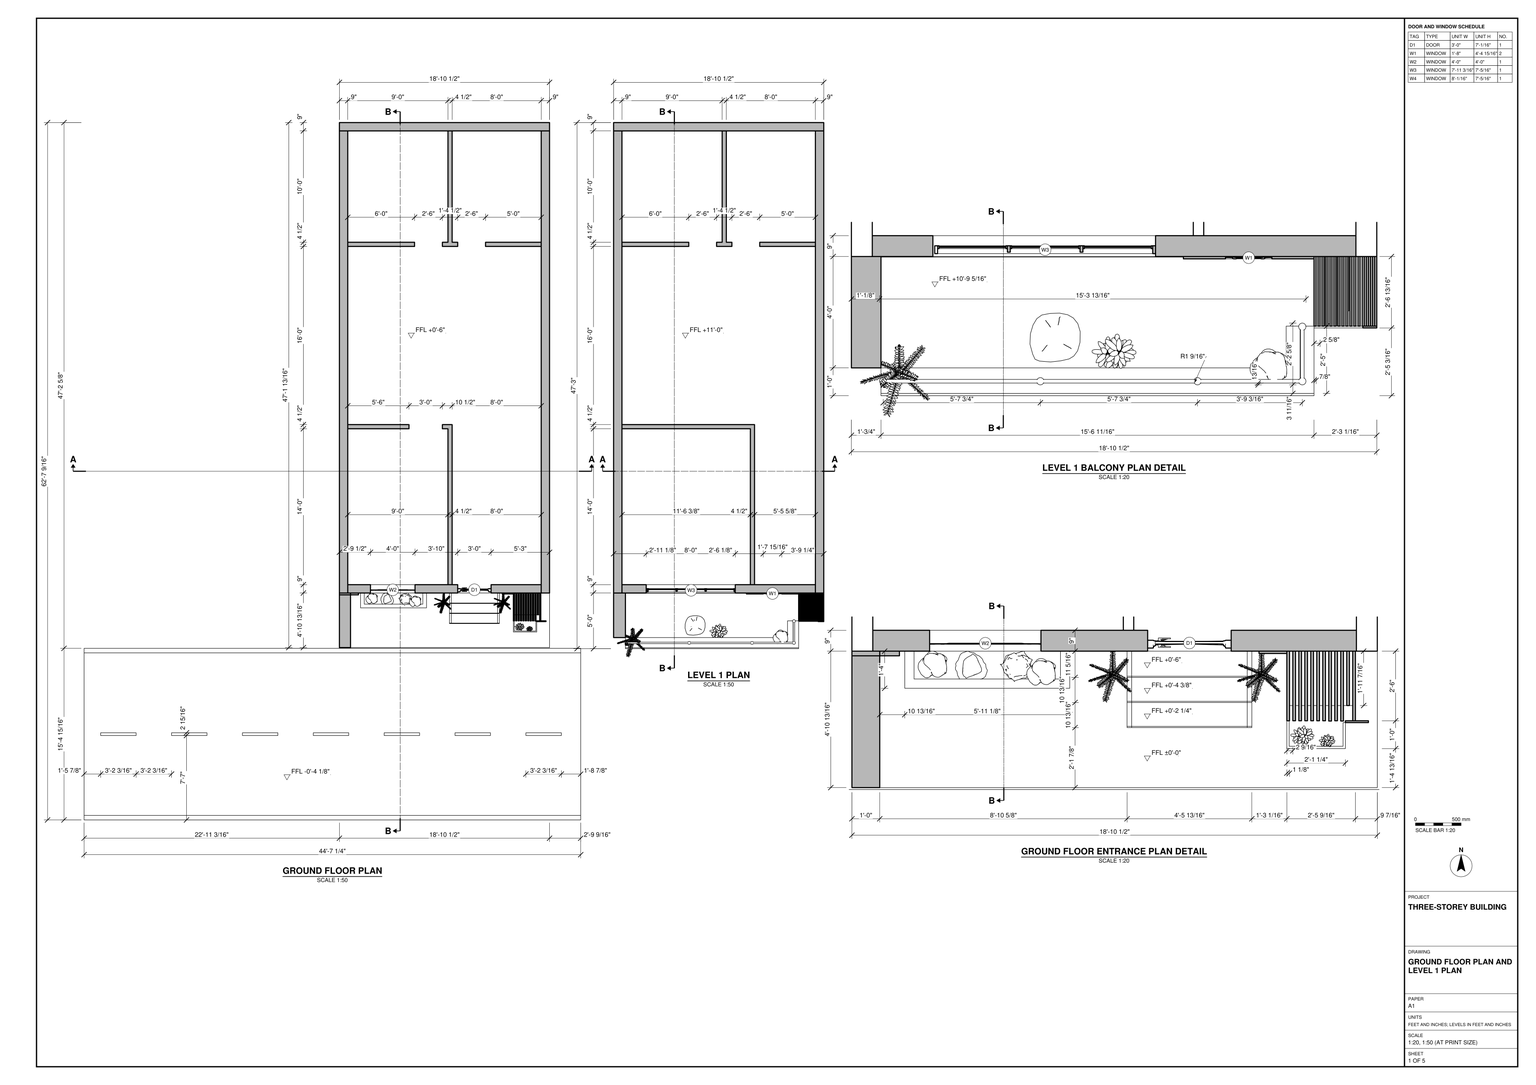
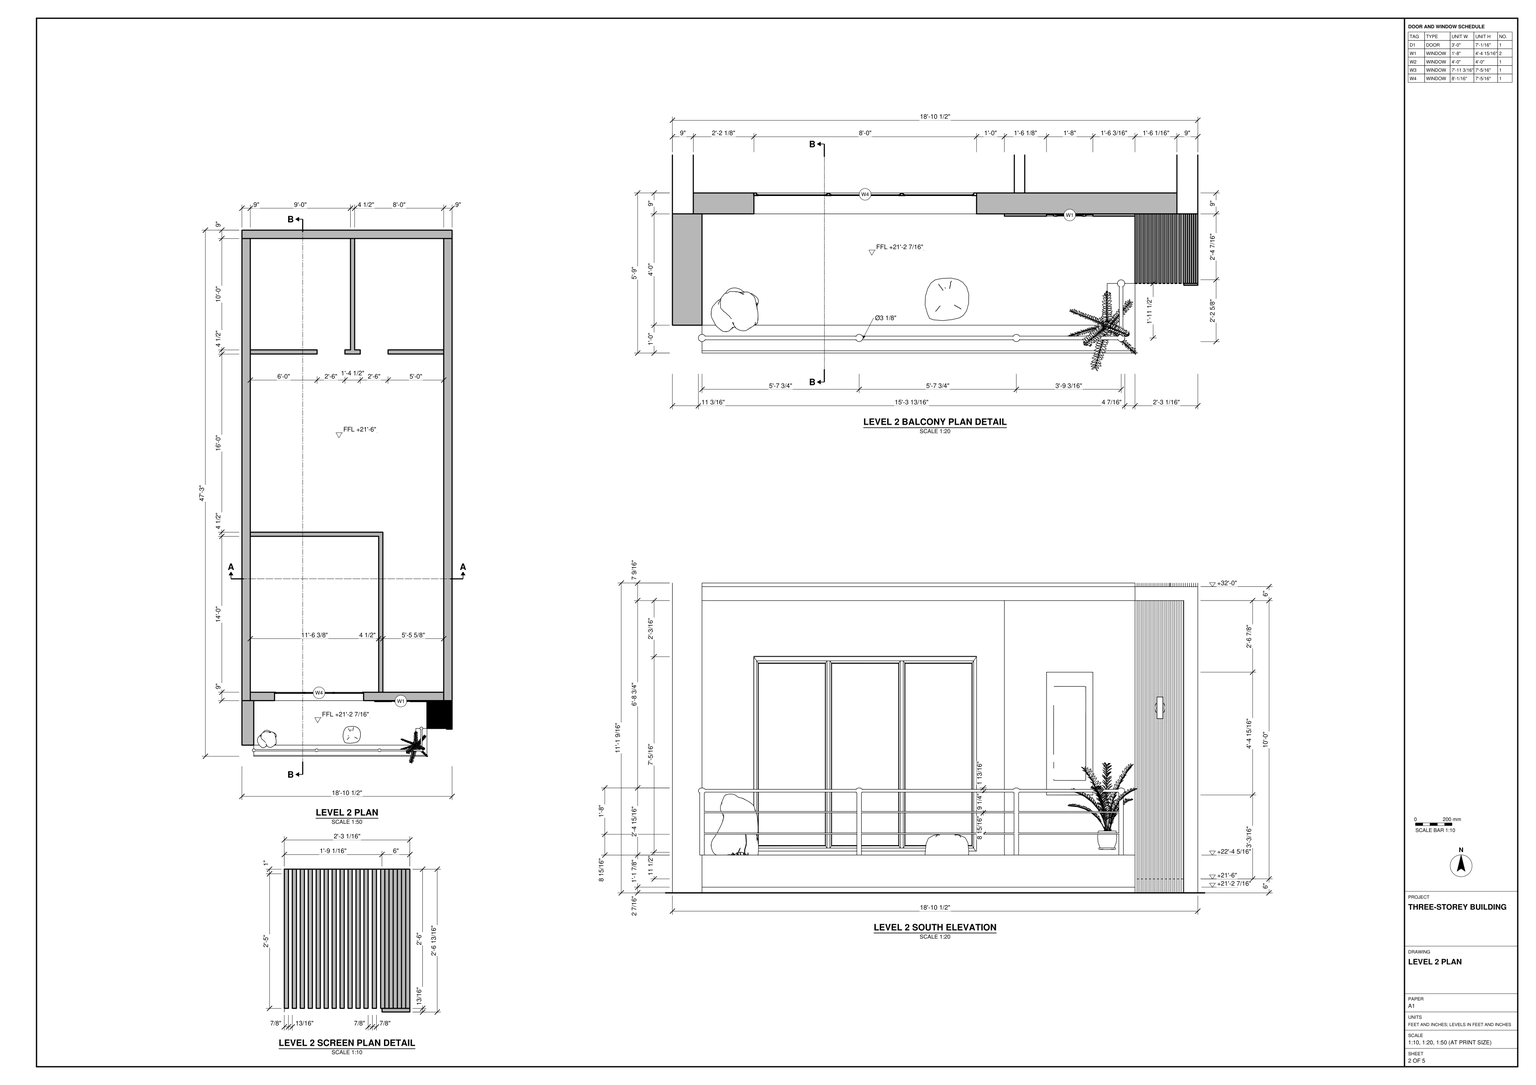
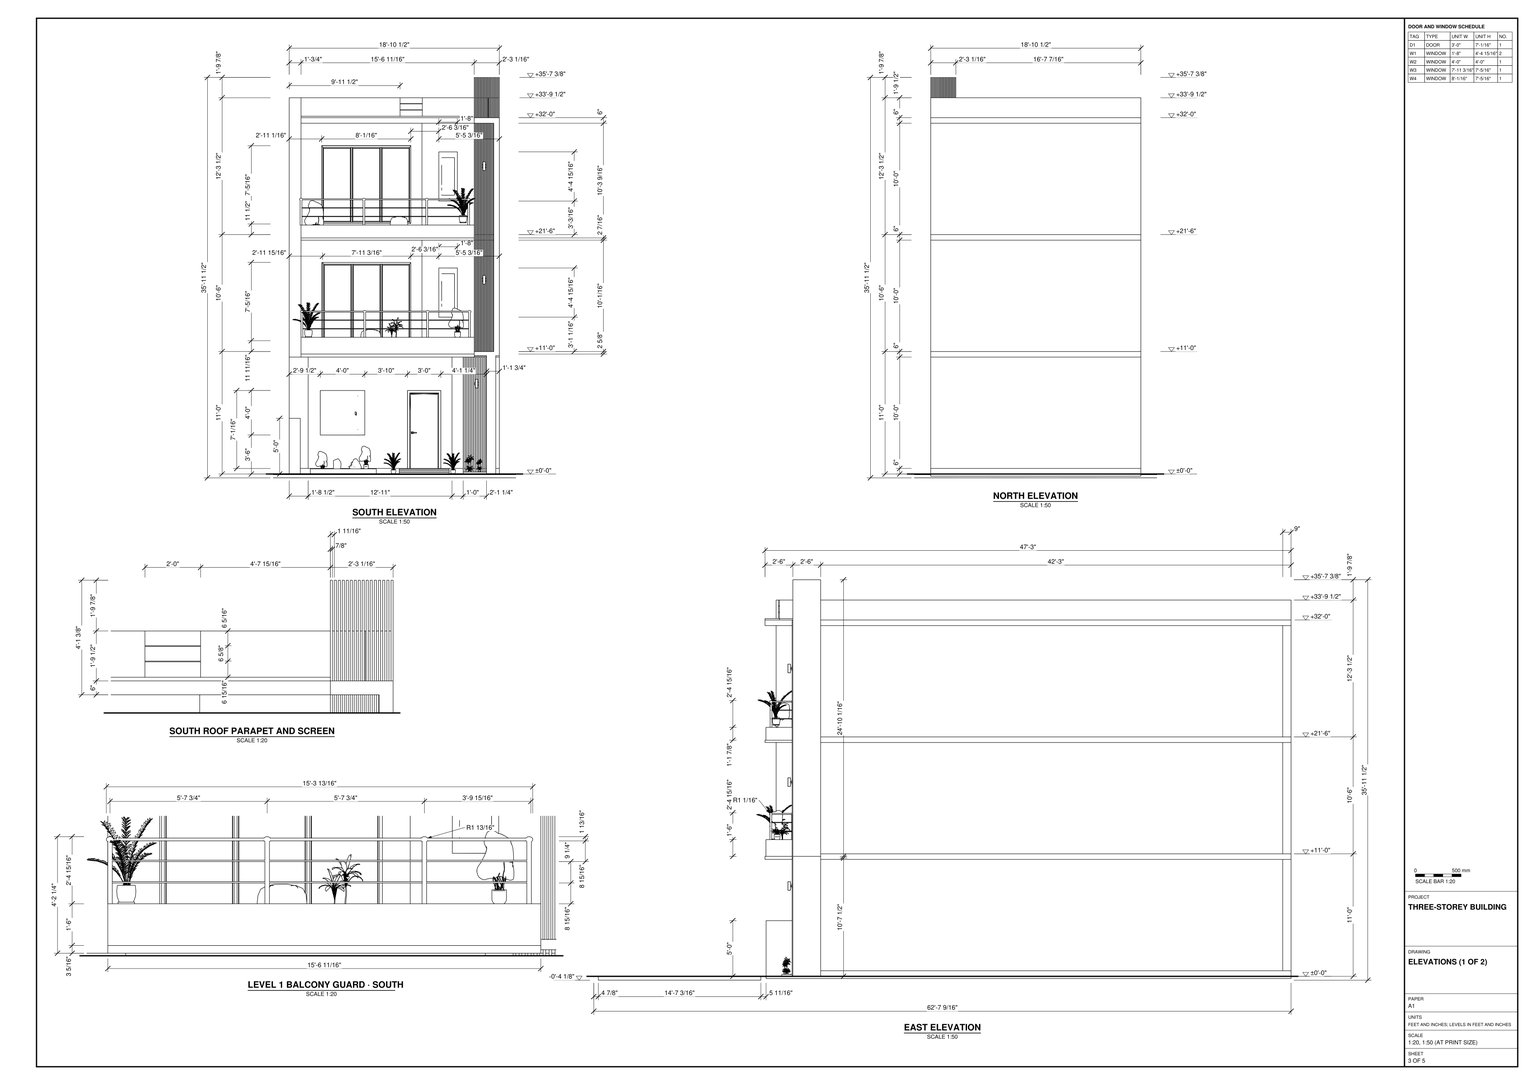
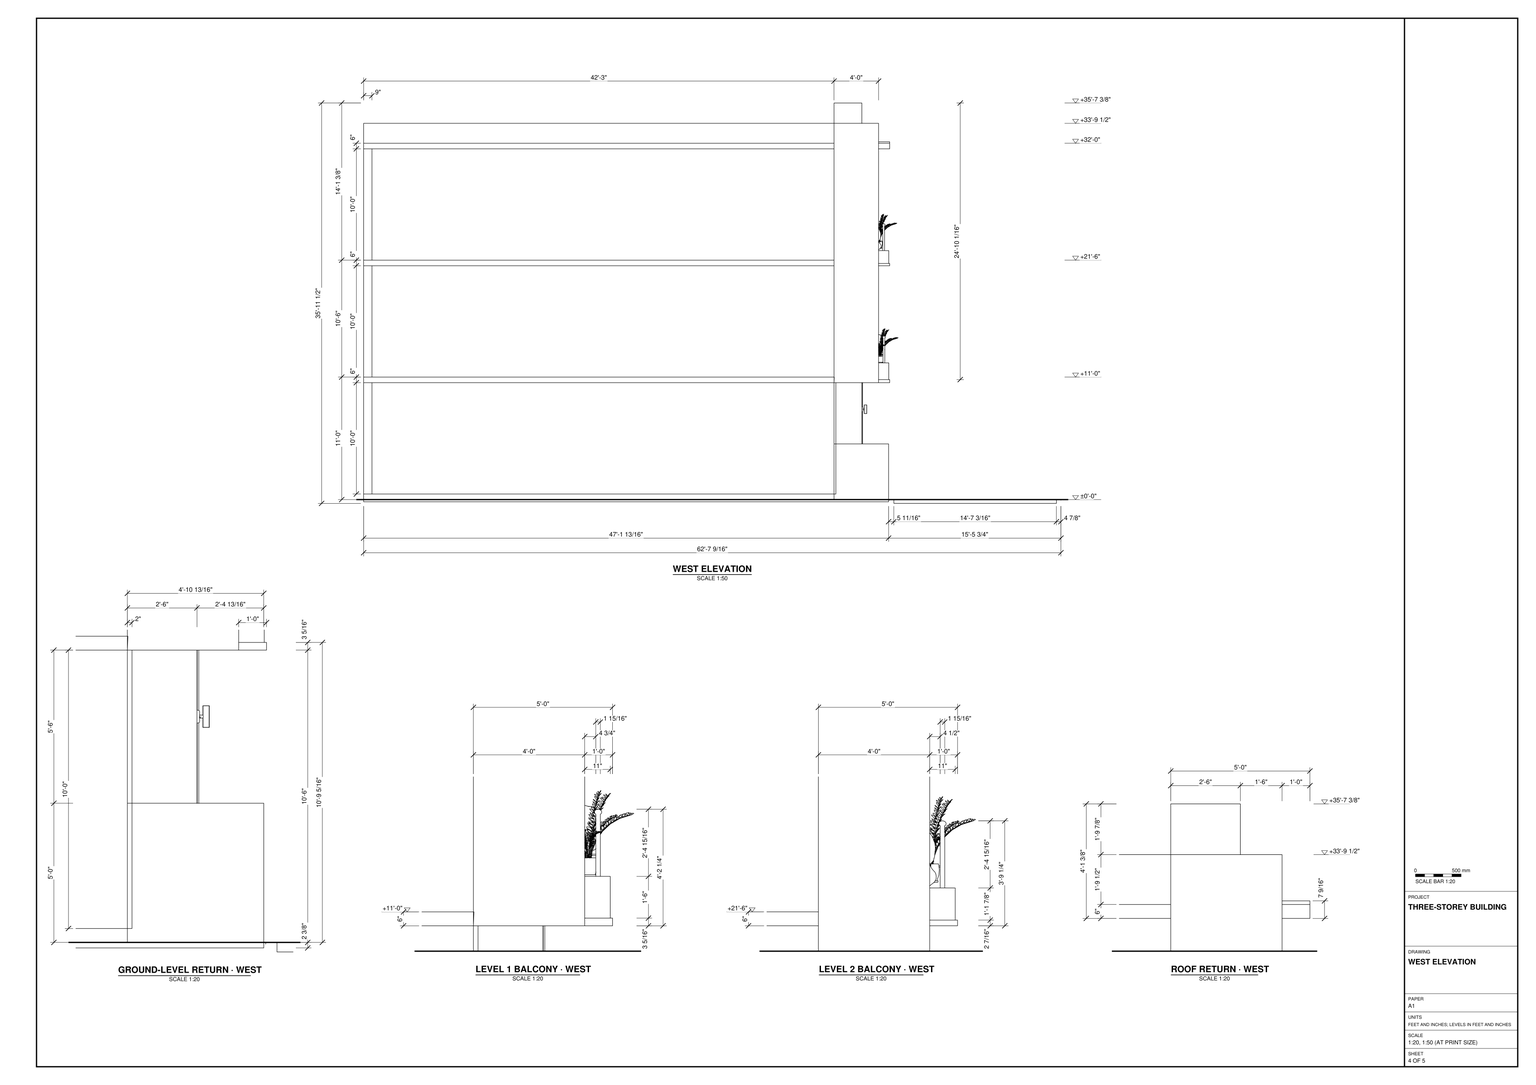
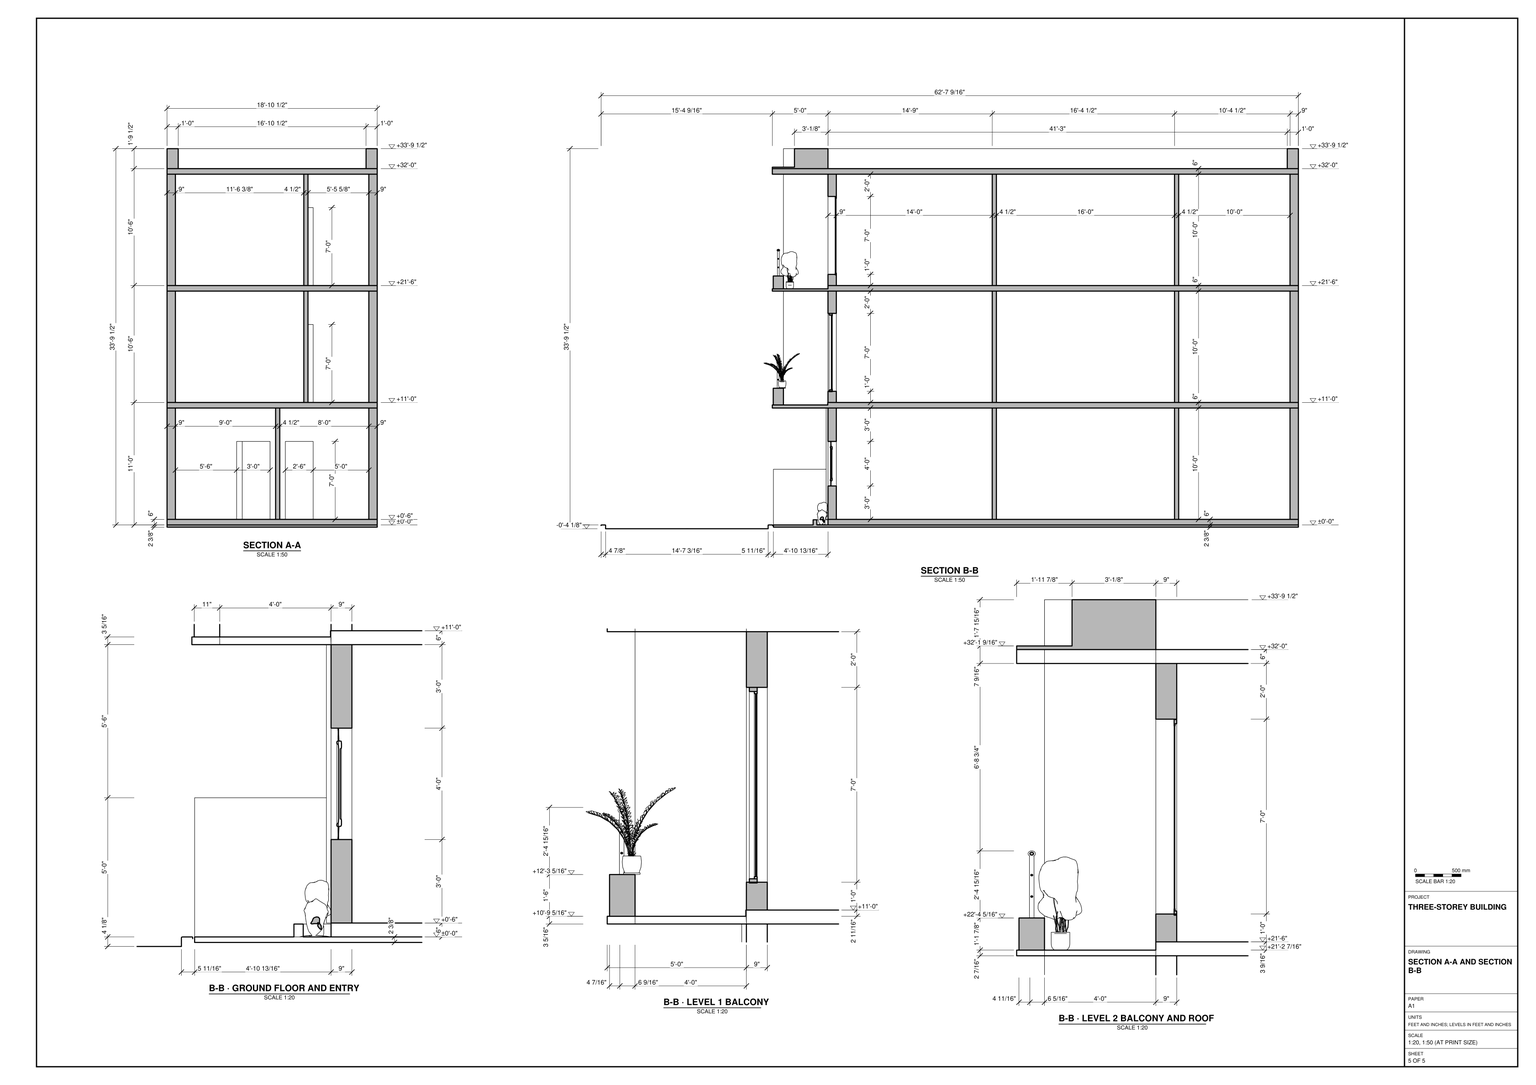
Use the five sheets in task_files/diagram_01.pdf to model the building and its front approach in SketchUp. Work in feet and inches. Including the approach and roof screen, the model shall measure 44'-7 1/4" across, 62'-7 9/16" from front to back and 35'-11 1/2" high. Use ±0'-0" as the ground datum, with Level 1 at +11'-0" and Level 2 at +21'-6".

Place the narrow building behind the wider approach as shown in the ground floor plan. Model the 9" exterior walls, 4 1/2" interior partitions and floor slabs. Follow each plan for the partition layout and the gaps connecting the rooms. At the south entrance, model the steps up to the door, the window to its left and the slatted screen to its right.

Build a balcony above the entrance at each upper level. Follow the balcony details for the slab edges, low solid guard bases, posts and horizontal rails. Set the wide glazed units and narrower windows behind the guards. Carry the upper slatted screen above the flat roof and reproduce its junction with the front parapet. Plants, lights and other loose or decorative items may be any suitable library components placed as shown.

Keep shell elements such as walls, slabs and roof, and each furniture or joinery piece, in separate groups or components. Use components for repeated parts. Save one SketchUp model as output_files/three_storey_building_with_stacked_south_balconies.skp.

# SketchUp Ruby script. Lengths in inches.
U = 1.inch
M = Sketchup.active_model
def pt(a) = Geom::Point3d.new(a.map { |v| v * U })
def face(e, loops, mat)
  f = e.add_face(loops[0].map { |a| pt(a) })
  loops[1..].each { |l| e.add_face(l.map { |a| pt(a) }).erase! }
  f.material = f.back_material = mat if mat
  f
end
# faces: each face lists its corners as indices into pts; further lists are holes
def faces(e, pts, list, mat = nil) = list.each { |f| face(e, (f[0].is_a?(Array) ? f : [f]).map { |l| l.map { |i| pts[i] } }, mat) }
# xy, xz, yz: faces in a plane at the given z, y or x. An outline is a flat list of corners, or four numbers for a rectangle; further outlines are holes
def ring(l) = l.size == 4 ? [[l[0], l[1]], [l[2], l[1]], [l[2], l[3]], [l[0], l[3]]] : l.each_slice(2).to_a
def flat(e, list, mat, &to3) = list.each { |f| face(e, (f[0].is_a?(Array) ? f : [f]).map { |l| ring(l).map { |u, v| to3.(u, v) } }, mat) }
def xy(e, z, list, mat = nil) = flat(e, list, mat) { |x, y| [x, y, z] }
def xz(e, y, list, mat = nil) = flat(e, list, mat) { |x, z| [x, y, z] }
def yz(e, x, list, mat = nil) = flat(e, list, mat) { |y, z| [x, y, z] }
def lines(e, pts, list) = list.each { |a, b| e.add_line(pt(pts[a]), pt(pts[b])) }
# prism: a flat outline (further loops are holes) pulled along v
def prism(e, loops, v, mat = nil)
  f = face(e, loops, mat); d = Geom::Vector3d.new(v.map { |x| x * U })
  f.pushpull(f.normal.samedirection?(d) ? d.length : -d.length)
end
def box(e, o, s, mat = nil) = prism(e, [[o, [o[0] + s[0], o[1], o[2]], [o[0] + s[0], o[1] + s[1], o[2]], [o[0], o[1] + s[1], o[2]]]], [0, 0, s[2]], mat)
def at(x, y, z, deg = 0) = Geom::Transformation.translation(pt([x, y, z])) * Geom::Transformation.rotation(ORIGIN, Z_AXIS, deg.degrees)
def axes(o, x, y, z) = Geom::Transformation.new([*x, 0, *y, 0, *z, 0, *pt(o).to_a, 1])
def part(name) = M.definitions.add(name)
# library, detail: a bought-in or finely detailed component or shape, given as its bounding box
def library(name, o, s) = part(name).tap { |d| box(d.entities, o, s) }
def detail(e, o, s) = box(e.add_group.entities, o, s)
def put(e, d, t, mat = nil) = e.add_instance(d, t).tap { |i| i.material = mat if mat }
def group(e, t, mat = nil) = e.add_group.tap { |g| g.transformation = t; g.material = mat if mat }.entities
root = M.entities
M.materials.add("Bricks A03 100cm").color = [95, 90, 86]
M.materials.add("Marble White 602 38.29cm").color = [255, 255, 255]
M.materials.add("Pearl Cream 2cm").color = [199, 183, 163]
M.materials.add("T8500 Silicone plaster D1 27.81cm").color = [255, 255, 255]
M.materials.add("Tiles B 130cm").color = [122, 119, 118]
M.materials.add("Tiles Marble Black 01 160cm").color = [32, 32, 32]
M.materials.add("Wall Paint Bumpy 01 Gray 100cm").color = [135, 135, 135]
M.materials.add("Wall Paint Dusk Blue Satin 300cm").color = [122, 143, 157]
M.materials.add("Wood Amboyan 13.2cm").color = [255, 255, 255]
M.materials.add("Wood Teak 33-35 100cm").color = [135, 81, 33]
c1 = library("Window 109 011",[-27.22,-3.26,-0.09],[54.45,6.58,70.7])
c2 = library("Window 46-47",[-61.02,-2.17,0],[122.04,4.34,74.02])
c3 = part("Vertical panel")
box(c3.entities,[0,0,-125.125],[0.9,30,298.0625],"Wood Amboyan 13.2cm")
c4 = part("Vertical panel \#2")
box(c4.entities,[0,-6.5625,0],[1.16,30,129.34],"Wood Amboyan 13.2cm")
c5 = part("Vertical panel \#1")
xy(c5.entities,0,[[0,-6.5625,1.16,23.4375]])
xy(c5.entities,125.9,[[0,-6.5625,1.16,23.4375]])
xz(c5.entities,-6.5625,[[0,0,1.16,125.9]],"Wood Amboyan 13.2cm")
xz(c5.entities,23.4375,[[0,0,1.16,125.9]])
yz(c5.entities,0,[[-6.5625,0,23.4375,125.9]])
yz(c5.entities,1.16,[[-6.5625,0,23.4375,125.9]])
c6 = part("Vertical panel \#3")
box(c6.entities,[0,-6.6875,0],[1.16,30.125,129.71],"Wood Amboyan 13.2cm")
c7 = part("Vertical panel \#4")
box(c7.entities,[0,-6.5625,0],[1.16,30,129.34],"Wood Amboyan 13.2cm")
c8 = part("Vertical panel \#5")
box(c8.entities,[0,-6.6875,0],[1.16,30.125,129.21],"Wood Amboyan 13.2cm")
c9 = part("Vertical panel \#6")
xy(c9.entities,0,[[0,0,1.16,23.4375]])
xy(c9.entities,129.21,[[0,0,1.16,23.4375]])
xz(c9.entities,0,[[0,0,1.16,129.21]],"Wood Amboyan 13.2cm")
xz(c9.entities,23.4375,[[0,0,1.16,129.21]])
yz(c9.entities,0,[[0,0,23.4375,129.21]])
yz(c9.entities,1.16,[[0,0,23.4375,129.21]])
c10 = part("Vertical panel \#7")
box(c10.entities,[0,-6.5625,0],[1.16,30,129.21])
c11 = part("Vertical panel assembly")
put(c11.entities,c7,at(0,0,0),"Wood Amboyan 13.2cm")
put(c11.entities,c8,at(2.58,0,0))
put(c11.entities,c9,at(5.16,0,0))
put(c11.entities,c10,at(7.75,0,0))
c12 = library("Door 243 065",[-19.36,-2.49,0],[38.72,4.98,81.96])
c13 = library("Sphere Light",[-3,-3,-3],[6,6,6])
c14 = library("Sphere Light\#2",[-3,-3,-3],[6,6,6])
c15 = library("Sphere Light\#3",[-3,-3,-3],[6,6,6])
c16 = library("Sphere Light\#4",[-3,-3,-3],[6,6,6])
c17 = library("Sphere Light\#5",[-3,-3,-3],[6,6,6])
c18 = library("Sphere Light\#6",[-3,-3,-3],[6,6,6])
c19 = library("Sphere Light\#7",[-3,-3,-3],[6,6,6])
c20 = library("Sphere Light\#8",[-3,-3,-3],[6,6,6])
c21 = library("Sphere Light\#9",[-3,-3,-3],[6,6,6])
c22 = library("Sphere Light\#10",[-3,-3,-3],[6,6,6])
c23 = library("Sphere Light\#11",[-3,-3,-3],[6,6,6])
c24 = library("Sphere Light\#12",[-3,-3,-3],[6,6,6])
c25 = part("Component\#12")
xy(c25.entities,0,[[0,0,53.8125,10.8125]])
xy(c25.entities,1.8125,[[0,-0.5,2,0],[2,-0.5,51.8125,0],[51.8125,-0.5,53.8125,0]])
xy(c25.entities,2.125,[[51.8125,-0.5,53.8125,10.8125]])
xy(c25.entities,2.125,[[0,-0.5,2,10.8125]],"Marble White 602 38.29cm")
xy(c25.entities,2.125,[[2,-0.5,51.8125,10.8125]],"Tiles Marble Black 01 160cm")
xz(c25.entities,-0.5,[[0,1.8125,53.8125,2.125]],"Marble White 602 38.29cm")
xz(c25.entities,0,[[0,0,53.8125,1.8125]],"Tiles Marble Black 01 160cm")
xz(c25.entities,10.8125,[[0,0,53.8125,2.125]])
yz(c25.entities,0,[[0,0,0,1.8125,-0.5,1.8125,-0.5,2.125,10.8125,2.125,10.8125,0]])
yz(c25.entities,53.8125,[[0,0,10.8125,0,10.8125,2.125,-0.5,2.125,-0.5,1.8125,0,1.8125]])
c26 = library("Potted Plant 02",[-16.98,-19.78,0],[30.04,38.68,37.52])
c27 = library("Potted Plant 13",[-10,-7.28,0],[18.93,15.17,39.22])
c28 = library("Indoor Plant 004",[-26.75,-21.09,0],[44.44,41.03,87.36])
c29 = library("Potted Plant 50-12",[-6.11,-5.26,0],[11.24,10.56,13.41])
c30 = library("Sedum Plant 66-24",[-7.97,-7.95,0.04],[16.42,16.31,19.57])
c31 = library("Climbing Plant 21-17",[-12.91,-12.55,0],[25.47,24.76,31.08])
c32 = library("Lamp Wall Outdoor 94-02",[-1.89,-4.65,-3.17],[3.78,4.65,6.35])
c33 = library("Spot Light",[-5.1,-5.1,-11.05],[10.2,10.2,11.05])
c34 = library("Spot Light\#1",[-5.1,-5.1,-11.05],[10.2,10.2,11.05])
c35 = library("Spot Light\#2",[-5.1,-5.1,-11.05],[10.2,10.2,11.05])
c36 = part("Group\#2")
box(c36.entities,[0,0,0],[226.5,9,120])
c37 = part("Group\#5")
xy(c37.entities,0,[[0,0,72,4.5],[102,0,102,4.5,108,4.5,108,124.5,112.5,124.5,112.5,4.5,118.5,4.5,118.5,0],[148.5,0,208.5,4.5]])
xy(c37.entities,84,[[72,0,102,4.5],[118.5,0,148.5,4.5]])
xy(c37.entities,120,[[0,0,208.5,0,208.5,4.5,112.5,4.5,112.5,124.5,108,124.5,108,4.5,0,4.5]])
xz(c37.entities,0,[[0,0,72,0,72,84,102,84,102,0,118.5,0,118.5,84,148.5,84,148.5,0,208.5,0,208.5,120,0,120]])
xz(c37.entities,4.5,[[0,0,0,120,108,120,108,0,102,0,102,84,72,84,72,0],[112.5,0,112.5,120,208.5,120,208.5,0,148.5,0,148.5,84,118.5,84,118.5,0]])
xz(c37.entities,124.5,[[108,0,112.5,120]])
yz(c37.entities,0,[[0,0,4.5,120]])
yz(c37.entities,72,[[0,0,4.5,84]])
yz(c37.entities,102,[[0,0,4.5,84]])
yz(c37.entities,108,[[4.5,0,124.5,120]])
yz(c37.entities,112.5,[[4.5,0,124.5,120]])
yz(c37.entities,118.5,[[0,0,4.5,84]])
yz(c37.entities,148.5,[[0,0,4.5,84]])
yz(c37.entities,208.5,[[0,0,4.5,120]])
c38 = part("Group\#4")
box(c38.entities,[0,0,0],[9,498,120])
c39 = part("Group\#11")
g1 = group(c39.entities,at(9,9,0))
prism(g1,[[[0,172.5,0],[142.89,172.5,0],[142.89,0,0],[138.39,0,0],[138.39,168.03,0],[0,168.03,0]]],[0,0,120])
g2 = group(c39.entities,at(9,0,0))
prism(g2,[[[208.5,9,0],[0,9,0],[0,9,120],[208.5,9,120]],[[26.125,9,96],[26.125,9,12],[122.125,9,12],[122.125,9,96]]],[0,-9,0])
put(c39.entities,c38,at(0,0,0))
put(c39.entities,c37,at(9,373.5,0))
g3 = group(c39.entities,at(217.5,0,0))
box(g3,[0,0,0],[9,498,120])
c40 = library("Group\#21",[0,0,0],[183.84,26.65,37.57])
c41 = library("Group\#26",[0,0,0],[256.85,486.62,4.11])
xy(root,-8.375,[[0,1.1875,226.5,567]])
xy(root,-6,[[[12,1.1875,226.5,1.1875,226.5,567,0,567,0,60,12,60],[22.78,44,22.78,60,26.78,60,26.78,48,89.91,48,89.91,60,93.91,60,93.91,44]]],"Tiles B 130cm")
xy(root,-5.9,[[187.5,18,187.5,30,188.5,30,188.5,19,211.73,19,211.73,29.21,212.73,29.21,212.73,18],[212.73,29.21,222.67,30],[200.41,30,201.57,60]])
xy(root,-3.9,[[187.5,18,212.73,18,212.73,29.21,211.73,29.21,211.73,19,188.5,19,188.5,30,187.5,30]])
xy(root,-0.4375,[[22.78,44,93.91,44,93.91,60,89.91,60,89.91,48,26.78,48,26.78,60,22.78,60]])
xy(root,0,[[175.5,59,187.5,60]])
xy(root,54,[[0,1.1875,12,60]],"T8500 Silicone plaster D1 27.81cm")
xy(root,120,[[0,12,12.75,60],[175.5,59,187.5,60]])
xy(root,121.5,[[199.4375,29.21,212.73,30],[222.67,29.21,226.5,30]])
xy(root,123.3125,[[200.41,30,201.57,60]])
xy(root,125.96,[[199.4375,29.21,220.5,30]])
xy(root,248.4375,[[12.75,1,199.4375,12],[187.4375,12,199.4375,30]],"Wall Paint Bumpy 01 Gray 100cm")
xy(root,262.3,[[12.75,1,199.4375,1,199.4375,30,193.4375,30,193.4375,6.5,12.75,6.5],[12.75,6.5,193.4375,6.5,193.4375,30,187.4375,30,187.4375,12,12.75,12]],"Wall Paint Bumpy 01 Gray 100cm")
xy(root,372,[[199.4375,29.21,220.5,30]])
xy(root,378,[[12.75,0,199.4375,15.5625],[12.75,15.5625,199.4375,60],[199.4375,29.21,226.5,30],[0,60,0,567,226.5,567,226.5,60,214.5,60,214.5,555,12,555,12,60]])
xy(root,379.5625,[[12.75,0,199.4375,0,199.4375,47,143.5,47,143.5,14.5625,119.5,14.5625,119.5,23.875,12.75,23.875],[119.5,14.5625,143.5,15.5625]])
xy(root,386.21,[[119.5,14.5625,143.5,15.5625]])
xy(root,386.52,[[119.5,14.5625,143.5,15.5625]])
xy(root,392.85,[[119.5,14.5625,143.5,15.5625]])
xy(root,393.17,[[119.5,14.5625,143.5,15.5625]])
xy(root,399.5,[[119.5,14.5625,143.5,15.5625],[119.5,15.5625,143.5,15.5625,143.5,47,199.4375,47,199.4375,60,12.75,60,12.75,23.875,119.5,23.875],[0,60,12,60,12,555,214.5,555,214.5,60,226.5,60,226.5,567,0,567]])
xy(root,399.5,[[0,12,12.75,60]],"Wall Paint Bumpy 01 Gray 100cm")
xz(root,0,[[12.75,378,199.4375,379.5625]])
xz(root,1,[[12.75,248.4375,199.4375,262.3]],"Wall Paint Bumpy 01 Gray 100cm")
xz(root,1.1875,[[0,-8.375,226.5,-8.375,226.5,-6,12,-6,12,54,0,54]],"Wall Paint Bumpy 01 Gray 100cm")
xz(root,12,[[0,120,12.75,399.5],[12.75,248.4375,187.4375,262.3]],"Wall Paint Bumpy 01 Gray 100cm")
xz(root,14.5625,[[119.5,379.5625,143.5,386.21],[119.5,386.52,143.5,392.85],[119.5,393.17,143.5,399.5]],"Wall Paint Dusk Blue Satin 300cm")
xz(root,15.5625,[[119.5,379.5625,143.5,386.21],[119.5,386.21,143.5,386.52],[119.5,386.52,143.5,392.85],[119.5,392.85,143.5,393.17],[119.5,393.17,143.5,399.5]])
xz(root,18,[[187.5,-5.9,212.73,-3.9]])
xz(root,19,[[188.5,-5.9,211.73,-3.9]])
xz(root,23.875,[[12.75,379.5625,119.5,399.5]],"Pearl Cream 2cm")
xz(root,29.21,[[211.73,-5.9,212.73,-3.9]])
xz(root,29.21,[[212.73,-5.9,222.67,-5.9,222.67,121.5,226.5,121.5,226.5,378,199.4375,378,199.4375,372,220.5,372,220.5,125.96,199.4375,125.96,199.4375,121.5,212.73,121.5]],"Wall Paint Bumpy 01 Gray 100cm")
xz(root,30,[[187.5,-5.9,188.5,-3.9],[212.73,-5.9,212.73,121.5,201.57,121.5,201.57,123.3125,200.41,123.3125,200.41,121.5,199.4375,121.5,199.4375,125.96,220.5,125.96,220.5,372,199.4375,372,199.4375,378,226.5,378,226.5,121.5,222.67,121.5,222.67,-5.9],[200.41,121.5,201.57,123.3125]])
xz(root,30,[[187.4375,248.4375,199.4375,262.3]],"Wall Paint Bumpy 01 Gray 100cm")
xz(root,30,[[200.41,-5.9,201.57,121.5]],"Wood Amboyan 13.2cm")
xz(root,44,[[22.78,-6,93.91,-0.4375]])
xz(root,47,[[143.5,379.5625,199.4375,399.5]],"Pearl Cream 2cm")
xz(root,48,[[26.78,-6,89.91,-0.4375]])
xz(root,59,[[175.5,0,187.5,120]],"Bricks A03 100cm")
xz(root,60,[[22.78,-6,26.78,-0.4375],[89.91,-6,93.91,-0.4375],[200.41,-5.9,201.57,123.3125],[175.5,0,187.5,120],[0,120,0,378,12,378,12,399.5,12.75,399.5,12.75,120],
  [0,378,12,399.5],[12.75,378,199.4375,399.5],[214.5,378,226.5,399.5]])
xz(root,60,[[0,-6,12,54]],"Tiles B 130cm")
xz(root,555,[[12,378,214.5,399.5]])
xz(root,567,[[0,-8.375,226.5,-6],[0,378,226.5,399.5]])
yz(root,0,[[1.1875,-8.375,1.1875,54,60,54,60,-6,567,-6,567,-8.375],[60,378,567,399.5]])
yz(root,0,[[12,120,60,399.5]],"Wall Paint Bumpy 01 Gray 100cm")
yz(root,12,[[60,378,555,399.5]])
yz(root,12,[[1.1875,-6,60,54]],"T8500 Silicone plaster D1 27.81cm")
yz(root,12.75,[[12,120,60,378],[0,378,12,379.5625],[12,378,15.5625,379.5625],[15.5625,378,60,378,60,399.5,23.875,399.5,23.875,379.5625,15.5625,379.5625],[12,379.5625,23.875,399.5]])
yz(root,12.75,[[1,248.4375,12,262.3]],"Wall Paint Bumpy 01 Gray 100cm")
yz(root,22.78,[[44,-6,60,-0.4375]])
yz(root,26.78,[[48,-6,60,-0.4375]])
yz(root,89.91,[[48,-6,60,-0.4375]])
yz(root,93.91,[[44,-6,60,-0.4375]])
yz(root,119.5,[[14.5625,379.5625,15.5625,386.21],[15.5625,379.5625,23.875,399.5],[14.5625,386.52,15.5625,392.85],[14.5625,393.17,15.5625,399.5]])
yz(root,143.5,[[14.5625,379.5625,15.5625,386.21],[15.5625,379.5625,47,399.5],[14.5625,386.52,15.5625,392.85],[14.5625,393.17,15.5625,399.5]])
yz(root,175.5,[[59,0,60,120]],"Bricks A03 100cm")
yz(root,187.4375,[[12,248.4375,30,262.3]],"Wall Paint Bumpy 01 Gray 100cm")
yz(root,187.5,[[18,-5.9,30,-3.9],[59,0,60,120]])
yz(root,188.5,[[19,-5.9,30,-3.9]])
yz(root,199.4375,[[29.21,121.5,30,125.96],[29.21,372,30,378],[0,378,15.5625,379.5625],[15.5625,378,60,378,60,399.5,47,399.5,47,379.5625,15.5625,379.5625]])
yz(root,199.4375,[[1,248.4375,30,262.3]],"Wall Paint Bumpy 01 Gray 100cm")
yz(root,200.41,[[30,-5.9,60,123.3125]],"Wood Amboyan 13.2cm")
yz(root,201.57,[[30,-5.9,60,123.3125]],"Wood Amboyan 13.2cm")
yz(root,211.73,[[19,-5.9,29.21,-3.9]])
yz(root,212.73,[[18,-5.9,29.21,-3.9],[29.21,-5.9,30,121.5]])
yz(root,214.5,[[60,378,555,399.5]])
yz(root,220.5,[[29.21,125.96,30,372]])
yz(root,222.67,[[29.21,-5.9,30,121.5]])
yz(root,226.5,[[1.1875,-8.375,567,-6],[29.21,121.5,30,378],[60,378,567,399.5]])
put(root,c1,axes([171.28,59.5,288.25],[0.36731,0,0],[0,-0.15202,0],[0,0,0.74878]))
put(root,c1,axes([171.28,59.5,163.13],[0.36731,0,0],[0,-0.15202,0],[0,0,0.74878]))
put(root,c2,axes([83.53,62.95,137.68],[0.78,0,0],[0,0.78,0],[0,0,1.13914]))
put(root,c2,axes([83.08,68.4375,263.5],[0.78726,0,0],[0,-0.25909,0],[0,0,1.13914]))
put(root,c3,at(199.4375,30,248.4375),"Wood Amboyan 13.2cm")
put(root,c3,at(201.15,30,248.4375))
put(root,c3,at(202.87,30,248.4375))
put(root,c3,at(204.59,30,248.4375))
put(root,c3,at(206.3,30,248.4375))
put(root,c3,at(208.02,30,248.4375))
put(root,c3,at(209.74,30,248.4375))
put(root,c3,at(211.45,30,248.4375))
put(root,c3,at(213.17,30,248.4375))
put(root,c3,at(214.89,30,248.4375))
put(root,c3,at(216.6,30,248.4375))
put(root,c3,at(218.4,30,248.4375))
put(root,c3,at(220.2,30,248.4375))
put(root,c3,at(222,30,248.4375))
put(root,c3,at(223.8,30,248.4375))
put(root,c3,at(225.6,30,248.4375))
put(root,c4,at(202.99,36.5625,-5.9))
put(root,c5,at(187.5,36.5625,-5.9),"Wood Amboyan 13.2cm")
put(root,c6,at(205.58,36.5625,-5.9))
put(root,c11,at(208.16,36.5625,-5.9))
put(root,c5,at(195.25,36.5625,-5.9),"Wood Amboyan 13.2cm")
put(root,c5,at(197.83,36.5625,-5.9))
put(root,c5,at(190.08,36.5625,-5.9),"Wood Amboyan 13.2cm")
put(root,c5,at(192.66,36.5625,-5.9),"Wood Amboyan 13.2cm")
put(root,c1,axes([57.5,63.4,36.06],[0.88154,0,0],[0,0.33,0],[0,0,0.67894]))
put(root,c12,axes([145.5,63.52,-0.07],[0.92977,0,0],[0,0.88,0],[0,0,1.02576]))
put(root,c13,at(32.11,30,372))
put(root,c14,at(175.65,30,372))
put(root,c15,at(137.11,30,372))
put(root,c16,at(85.03,30,372))
put(root,c17,at(32.23,30,246))
put(root,c18,at(85.22,30,246))
put(root,c19,at(137.14,30,246))
put(root,c20,at(175.66,30,246))
put(root,c21,at(32.28,30,118))
put(root,c22,at(84.97,30,118))
put(root,c23,at(136.62,30,120))
put(root,c24,at(178.0625,30,120))
put(root,c25,at(118.61,49.1875,-2.125))
put(root,c25,at(118.61,38.375,-3.75))
put(root,c25,at(118.61,27.5625,-5.875))
put(root,c26,axes([176.64,50.15,-6],[0.62,0,0],[0,0.62,0],[0,0,0.62]))
put(root,c26,axes([112.46,50.15,-6],[0.62,0,0],[0,0.62,0],[0,0,0.62]))
put(root,c27,axes([194.46,23.62,-6],[0.53,0,0],[0,0.53,0],[0,0,0.53]))
put(root,c27,axes([205.04,21.35,-3.9],[0.36,0,0],[0,0.36,0],[0,0,0.36]))
put(root,c28,axes([36.02,54.42,-6],[0.28,0,0],[0,0.28,0],[0,0,0.28]))
put(root,c28,axes([82.85,51.25,-0.4375],[0.28,0,0],[0,0.28,0],[0,0,0.28]))
put(root,c29,axes([71.5,53.43,-6],[1.24,0,0],[0,1.24,0],[0,0,1.24]))
put(root,c26,at(20.73,10.61,141.3125))
put(root,c26,at(187.4375,12,264.68))
put(root,c30,axes([51.3,52.98,-6.03],[0.84,0,0],[0,0.84,0],[0,0,0.84]))
put(root,c27,at(113.76,18.66,123.3125))
put(root,c31,axes([87.95,25.23,123.3125],[0.8505,0,0],[0,0.8505,0],[0,0,0.8505]))
put(root,c31,axes([118.48,23.27,248.4375],[0.74,0,0],[0,0.74,0],[0,0,0.74]))
put(root,c28,axes([181.48,12.99,141.3125],[0.36,0,0],[0,0.36,0],[0,0,0.36]))
put(root,c28,axes([28.98,18.9,248.4375],[0.46,0,0],[0,0.46,0],[0,0,0.46]))
put(root,c32,axes([201.98,30,91.35],[1.15,0,0],[0,1.15,0],[0,0,1.472]))
put(root,c32,axes([210.18,30,203.3],[1.15,0,0],[0,1.15,0],[0,0,1.472]))
put(root,c32,axes([210.18,30,325.77],[1.15,0,0],[0,1.15,0],[0,0,1.472]))
put(root,c33,at(210.29,26.29,321.13))
put(root,c34,at(210.19,26.45,198.67))
put(root,c35,at(201.94,26.85,86.71))
put(root,c34,axes([210.18,27.36,207.07],[1,0,0],[0,1,0],[0,0,-1]))
put(root,c34,axes([201.37,26.97,95.12],[1,0,0],[0,1,0],[0,0,-1]))
g4 = group(root,at(0,60,-6))
box(g4,[0,0,0],[226.5,507,6])
put(root,c36,at(0,558,0))
g5 = group(root,at(217.5,60,0))
box(g5,[0,0,0],[9,498,120])
put(root,c37,at(9,433.5,0))
g6 = group(root,at(9,69,0))
xy(g6,0,[[108,0,108,168,102,168,102,172.5,112.5,172.5,112.5,0],[0,168,66,172.5]])
xy(g6,84,[[66,168,102,172.5]])
xy(g6,120,[[108,0,112.5,0,112.5,172.5,0,172.5,0,168,108,168]])
xz(g6,0,[[108,0,112.5,120]])
xz(g6,168,[[0,0,66,0,66,84,102,84,102,0,108,0,108,120,0,120]])
xz(g6,172.5,[[0,0,0,120,112.5,120,112.5,0,102,0,102,84,66,84,66,0]])
yz(g6,0,[[168,0,172.5,120]])
yz(g6,66,[[168,0,172.5,84]])
yz(g6,102,[[168,0,172.5,84]])
yz(g6,108,[[0,0,168,120]])
yz(g6,112.5,[[0,0,172.5,120]])
g7 = group(root,at(0,60,120))
xy(g7,0,[[0,0,226.5,507]])
xy(g7,0,[[12.75,-60,199.4375,0]],"Wood Teak 33-35 100cm")
xy(g7,3.3125,[[12.75,-60,199.4375,-0.23]])
xy(g7,6,[[0,-0.23,199.4375,-0.23,199.4375,0,226.5,0,226.5,507,0,507]])
xz(g7,-60,[[12.75,0,199.4375,3.3125]])
xz(g7,-0.23,[[12.75,3.3125,199.4375,6]])
xz(g7,0,[[199.4375,0,226.5,6]])
xz(g7,507,[[0,0,226.5,6]])
yz(g7,0,[[0,0,-0.23,6,507,6,507,0]])
yz(g7,12.75,[[-60,0,-60,3.3125,-0.23,3.3125,-0.23,6,0,0]])
yz(g7,199.4375,[[-60,0,0,0,0,6,-0.23,6,-0.23,3.3125,-60,3.3125]])
yz(g7,226.5,[[0,0,507,6]])
p = [[0,-0.23,6],[0,0,0],[12.75,0,0],[12.75,-0.23,6]]
faces(g7,p,[[0,1,2,3]])
g8 = group(root,at(0,60,126))
put(g8,c39,at(0,0,0))
put(g8,c36,at(0,498,0))
g9 = group(root,at(0,60,252))
put(g9,c39,at(0,0,0))
put(g9,c36,at(0,498,0))
g10 = group(root,at(0,60,246))
xy(g10,0,[[12.75,-60,12.75,0,0,0,0,507,226.5,507,226.5,0,199.4375,0,199.4375,-60]],"Wood Teak 33-35 100cm")
xy(g10,2.4375,[[12.75,-60,199.4375,0]])
xy(g10,6,[[0,0,226.5,507]])
xz(g10,-60,[[12.75,0,199.4375,2.4375]])
xz(g10,0,[[0,0,12.75,6],[199.4375,0,226.5,6],[12.75,2.4375,199.4375,6]])
xz(g10,507,[[0,0,226.5,6]])
yz(g10,0,[[0,0,507,6]])
yz(g10,12.75,[[-60,0,0,2.4375]])
yz(g10,199.4375,[[-60,0,0,2.4375]])
yz(g10,226.5,[[0,0,507,6]])
g11 = group(root,at(0,60,372))
xy(g11,0,[[12.75,-60,12.75,0,0,0,0,507,226.5,507,226.5,0,199.4375,0,199.4375,-60]],"Wood Teak 33-35 100cm")
xy(g11,6,[[12.75,-60,199.4375,-60,199.4375,0,226.5,0,226.5,507,0,507,0,0,12.75,0]])
xz(g11,-60,[[12.75,0,199.4375,6]])
xz(g11,0,[[0,0,12.75,6],[199.4375,0,226.5,6]])
xz(g11,507,[[0,0,226.5,6]])
yz(g11,0,[[0,0,507,6]])
yz(g11,12.75,[[-60,0,0,6]])
yz(g11,199.4375,[[-60,0,0,6]])
yz(g11,226.5,[[0,0,507,6]])
g12 = group(root,at(143.125,59,248.4375))
xy(g12,0,[[0,0,56.3125,1]])
xy(g12,39.75,[[18.16,0,38.16,1]])
xy(g12,92.6875,[[18.16,0,38.16,1]])
xy(g12,123.5625,[[0,0,56.3125,1]])
xz(g12,0,[[[0,0,56.3125,123.5625],[18.16,39.75,38.16,92.6875]]],"Bricks A03 100cm")
xz(g12,1,[[[0,0,56.3125,123.5625],[18.16,39.75,38.16,92.6875]]])
yz(g12,0,[[0,0,1,123.5625]],"Bricks A03 100cm")
yz(g12,18.16,[[0,39.75,1,92.6875]])
yz(g12,38.16,[[0,39.75,1,92.6875]])
yz(g12,56.3125,[[0,0,1,123.5625]])
g13 = group(root,at(143.125,59,123.3125))
prism(g13,[[[0,1,0],[0,1,123.5625],[56.3125,1,123.5625],[56.3125,1,0]],[[18.16,1,92.6875],[18.16,1,39.75],[38.16,1,39.75],[38.16,1,92.6875]]],[0,-1,0],"Bricks A03 100cm")
g14 = group(root,at(187.5,36.5625,-6))
box(g14,[0,0,0],[29.5625,23.4375,0.1])
g15 = group(root,at(12.75,0,123.3125))
xy(g15,0,[[0,1,0,12,174.6875,12,174.6875,30,186.6875,30,186.6875,1]],"Wall Paint Bumpy 01 Gray 100cm")
xy(g15,18,[[0,1,186.6875,1,186.6875,30,180.6875,30,180.6875,6.5,0,6.5],[0,6.5,180.6875,6.5,180.6875,30,174.6875,30,174.6875,12,0,12]],"Wall Paint Bumpy 01 Gray 100cm")
xz(g15,1,[[0,0,186.6875,18]],"Wall Paint Bumpy 01 Gray 100cm")
xz(g15,12,[[0,0,174.6875,18]],"Wall Paint Bumpy 01 Gray 100cm")
xz(g15,30,[[174.6875,0,186.6875,18]],"Wall Paint Bumpy 01 Gray 100cm")
yz(g15,0,[[1,0,12,18]],"Wall Paint Bumpy 01 Gray 100cm")
yz(g15,174.6875,[[12,0,30,18]],"Wall Paint Bumpy 01 Gray 100cm")
yz(g15,186.6875,[[1,0,30,18]],"Wall Paint Bumpy 01 Gray 100cm")
put(root,c40,axes([11.18,4.93,262.3],[1,0,0],[0,1,0],[0,0,0.77]))
put(root,c40,axes([12.125,4.67,141.3125],[1,0,0],[0,1,0],[0,0,0.77]))
g16 = group(root,at(0,60,0))
g17 = group(g16,at(0,0,0))
g18 = group(g17,at(9,0,0))
xy(g18,0,[[0,0,118.5,9],[154.5,0,208.5,9]])
xy(g18,36,[[24.5,0,72.5,9]])
xy(g18,84,[[24.5,0,72.5,9],[118.5,0,154.5,9]])
xy(g18,120,[[0,0,208.5,9]])
xz(g18,0,[[-9,0,0,120],[[0,0,118.5,0,118.5,84,154.5,84,154.5,0,208.5,0,208.5,120,0,120],[24.5,36,72.5,84]]])
xz(g18,9,[[[0,0,0,120,208.5,120,208.5,0,154.5,0,154.5,84,118.5,84,118.5,0],[24.5,36,72.5,84]]])
yz(g18,0,[[0,0,9,120]])
yz(g18,24.5,[[0,36,9,84]])
yz(g18,72.5,[[0,36,9,84]])
yz(g18,118.5,[[0,0,9,84]])
yz(g18,154.5,[[0,0,9,84]])
yz(g18,208.5,[[0,0,9,120]])
put(g17,c38,at(0,0,0))
g19 = group(g16,at(0,-2,0))
xy(g19,0,[[0,0,20.49,2]])
xy(g19,120,[[0,0,20.49,2]])
xz(g19,0,[[0,0,20.49,120]],"Wall Paint Bumpy 01 Gray 100cm")
xz(g19,2,[[0,0,20.49,120]])
yz(g19,0,[[0,0,2,120]])
yz(g19,20.49,[[0,0,2,120]])
put(root,c41,axes([-275.19,0.36,-10.11],[0,-0.72,0],[1.1,0,0],[0,0,1]))
